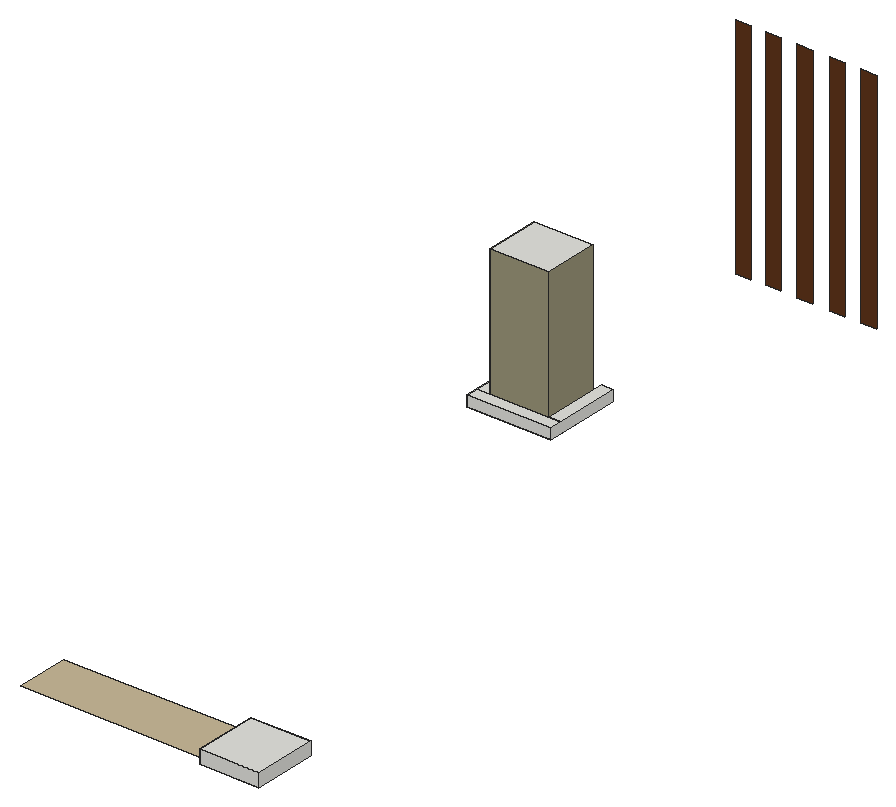
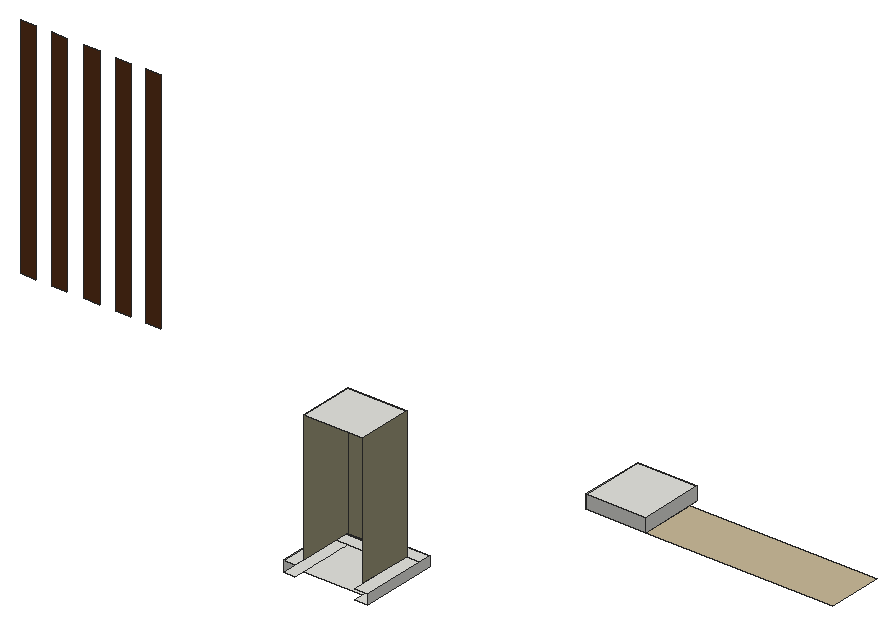
# SketchUp Ruby script. Lengths in inches.
U = 1.inch
M = Sketchup.active_model
def pt(a) = Geom::Point3d.new(a.map { |v| v * U })
def face(e, loops, mat)
  f = e.add_face(loops[0].map { |a| pt(a) })
  loops[1..].each { |l| e.add_face(l.map { |a| pt(a) }).erase! }
  f.material = f.back_material = mat if mat
  f
end
# faces: each face lists its corners as indices into pts; further lists are holes
def faces(e, pts, list, mat = nil) = list.each { |f| face(e, (f[0].is_a?(Array) ? f : [f]).map { |l| l.map { |i| pts[i] } }, mat) }
# xy, xz, yz: faces in a plane at the given z, y or x. An outline is a flat list of corners, or four numbers for a rectangle; further outlines are holes
def ring(l) = l.size == 4 ? [[l[0], l[1]], [l[2], l[1]], [l[2], l[3]], [l[0], l[3]]] : l.each_slice(2).to_a
def flat(e, list, mat, &to3) = list.each { |f| face(e, (f[0].is_a?(Array) ? f : [f]).map { |l| ring(l).map { |u, v| to3.(u, v) } }, mat) }
def xy(e, z, list, mat = nil) = flat(e, list, mat) { |x, y| [x, y, z] }
def xz(e, y, list, mat = nil) = flat(e, list, mat) { |x, z| [x, y, z] }
def yz(e, x, list, mat = nil) = flat(e, list, mat) { |y, z| [x, y, z] }
def lines(e, pts, list) = list.each { |a, b| e.add_line(pt(pts[a]), pt(pts[b])) }
# prism: a flat outline (further loops are holes) pulled along v
def prism(e, loops, v, mat = nil)
  f = face(e, loops, mat); d = Geom::Vector3d.new(v.map { |x| x * U })
  f.pushpull(f.normal.samedirection?(d) ? d.length : -d.length)
end
def box(e, o, s, mat = nil) = prism(e, [[o, [o[0] + s[0], o[1], o[2]], [o[0] + s[0], o[1] + s[1], o[2]], [o[0], o[1] + s[1], o[2]]]], [0, 0, s[2]], mat)
def at(x, y, z, deg = 0) = Geom::Transformation.translation(pt([x, y, z])) * Geom::Transformation.rotation(ORIGIN, Z_AXIS, deg.degrees)
def axes(o, x, y, z) = Geom::Transformation.new([*x, 0, *y, 0, *z, 0, *pt(o).to_a, 1])
def part(name) = M.definitions.add(name)
# library, detail: a bought-in or finely detailed component or shape, given as its bounding box
def library(name, o, s) = part(name).tap { |d| box(d.entities, o, s) }
def detail(e, o, s) = box(e.add_group.entities, o, s)
def put(e, d, t, mat = nil) = e.add_instance(d, t).tap { |i| i.material = mat if mat }
def group(e, t, mat = nil) = e.add_group.tap { |g| g.transformation = t; g.material = mat if mat }.entities
root = M.entities
M.materials.add("[Quartz Light Brown]").color = [199, 184, 152]
M.materials.add("[Stone Coursed Rough]").color = [155, 150, 122]
M.materials.add("[Wood Cherry Original]").color = [94, 53, 26]
xy(root,57.8125,[[65.07,93.68,81.17,96.24],[65.07,96.24,66.82,111],[66.82,96.24,79.1,111],[79.1,96.24,81.17,111]])
xy(root,57.8125,[[14.76,96.24,65.07,111]],"[Quartz Light Brown]")
xy(root,61.4375,[[65.07,93.68,81.17,111]])
xy(root,93.02,[[52.21,199.92,74.94,203.17],[52.21,203.17,55.77,220.79],[55.77,203.17,71.76,217.98],[71.76,203.17,74.94,220.79]])
xy(root,95.8,[[52.21,199.92,74.94,203.17],[52.21,203.17,55.77,220.79]])
xy(root,95.87,[[71.76,203.17,74.94,220.79]])
xy(root,130.875,[[55.77,203.17,71.76,217.98]])
xz(root,93.68,[[65.07,57.8125,81.17,61.4375]])
xz(root,111,[[65.07,57.8125,81.17,61.4375]])
xz(root,199.92,[[52.21,93.02,74.94,95.8]])
xz(root,203.17,[[55.77,95.8,74.94,95.8,74.94,95.87,71.76,95.87,71.76,130.875,55.77,130.875]],"[Stone Coursed Rough]")
xz(root,217.51,[[110.6,137.875,114.76,199.07],[118.6,137.875,122.76,199.07],[127.16,137.875,131.32,199.07],[135.85,137.875,140.01,199.07],[144.35,137.875,148.51,199.07]],"[Wood Cherry Original]")
yz(root,52.21,[[199.92,93.02,220.79,95.8]])
yz(root,55.77,[[203.17,95.8,217.98,130.875]],"[Stone Coursed Rough]")
yz(root,65.07,[[93.68,57.8125,111,61.4375]])
yz(root,71.76,[[203.17,95.87,217.98,130.875]],"[Stone Coursed Rough]")
yz(root,74.94,[[199.92,93.02,220.79,93.02,220.79,95.87,203.17,95.87,203.17,95.8,199.92,95.8]])
yz(root,81.17,[[93.68,57.8125,111,61.4375]])
